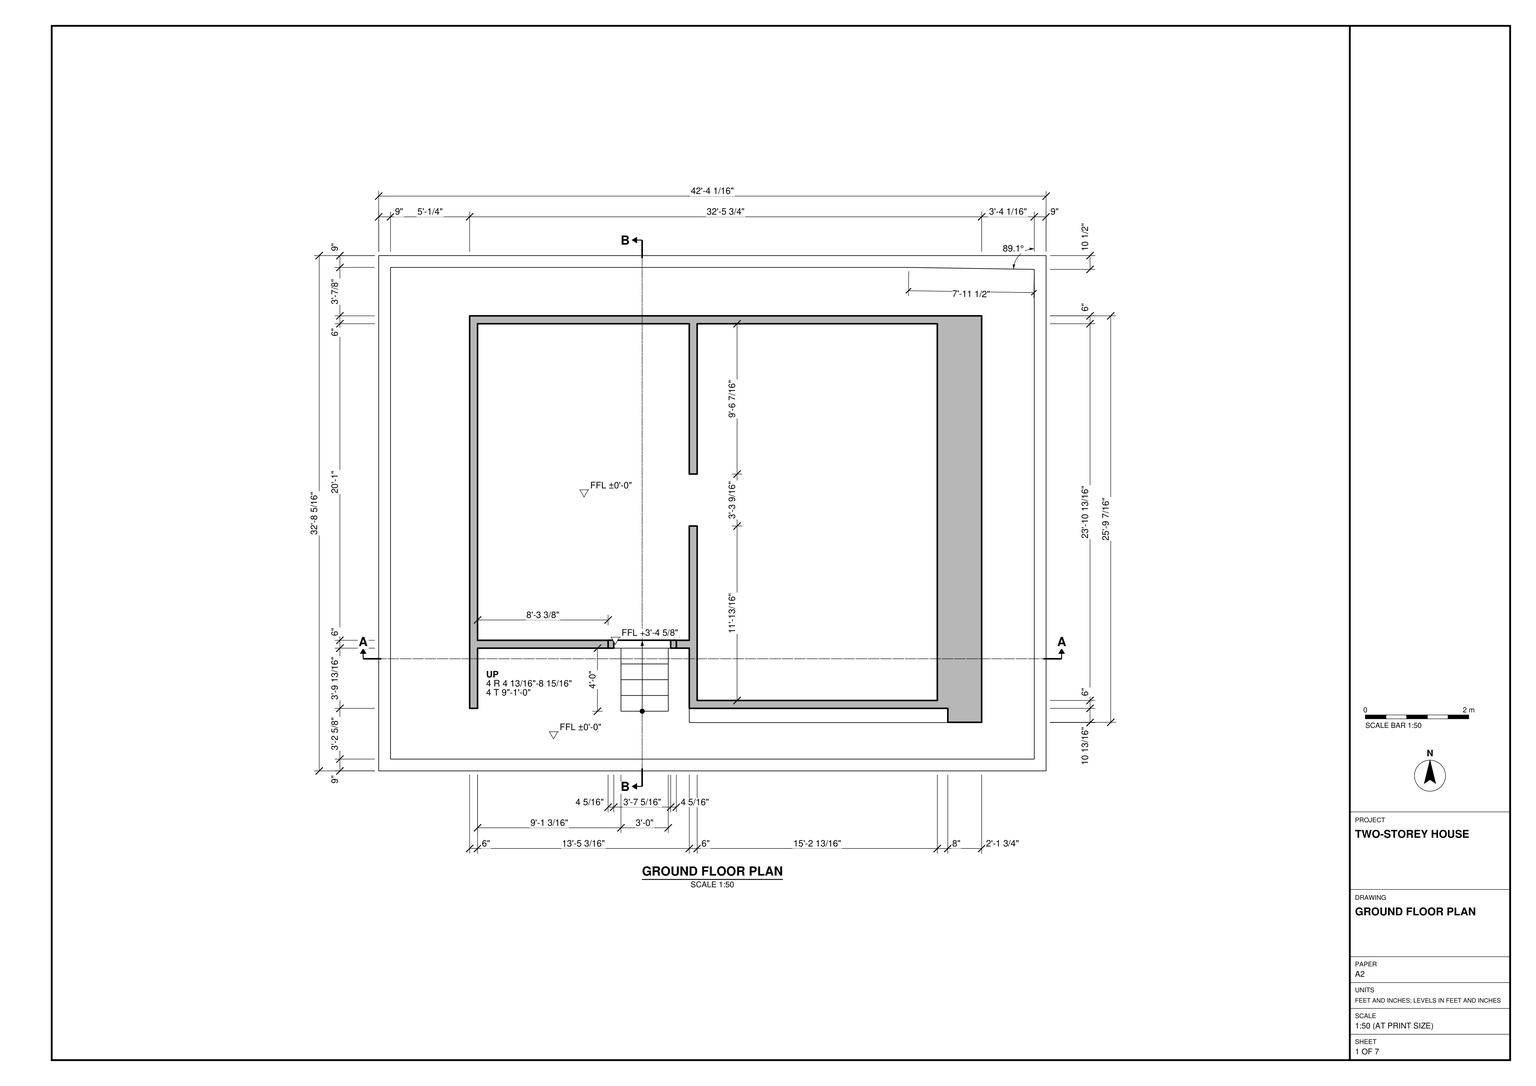
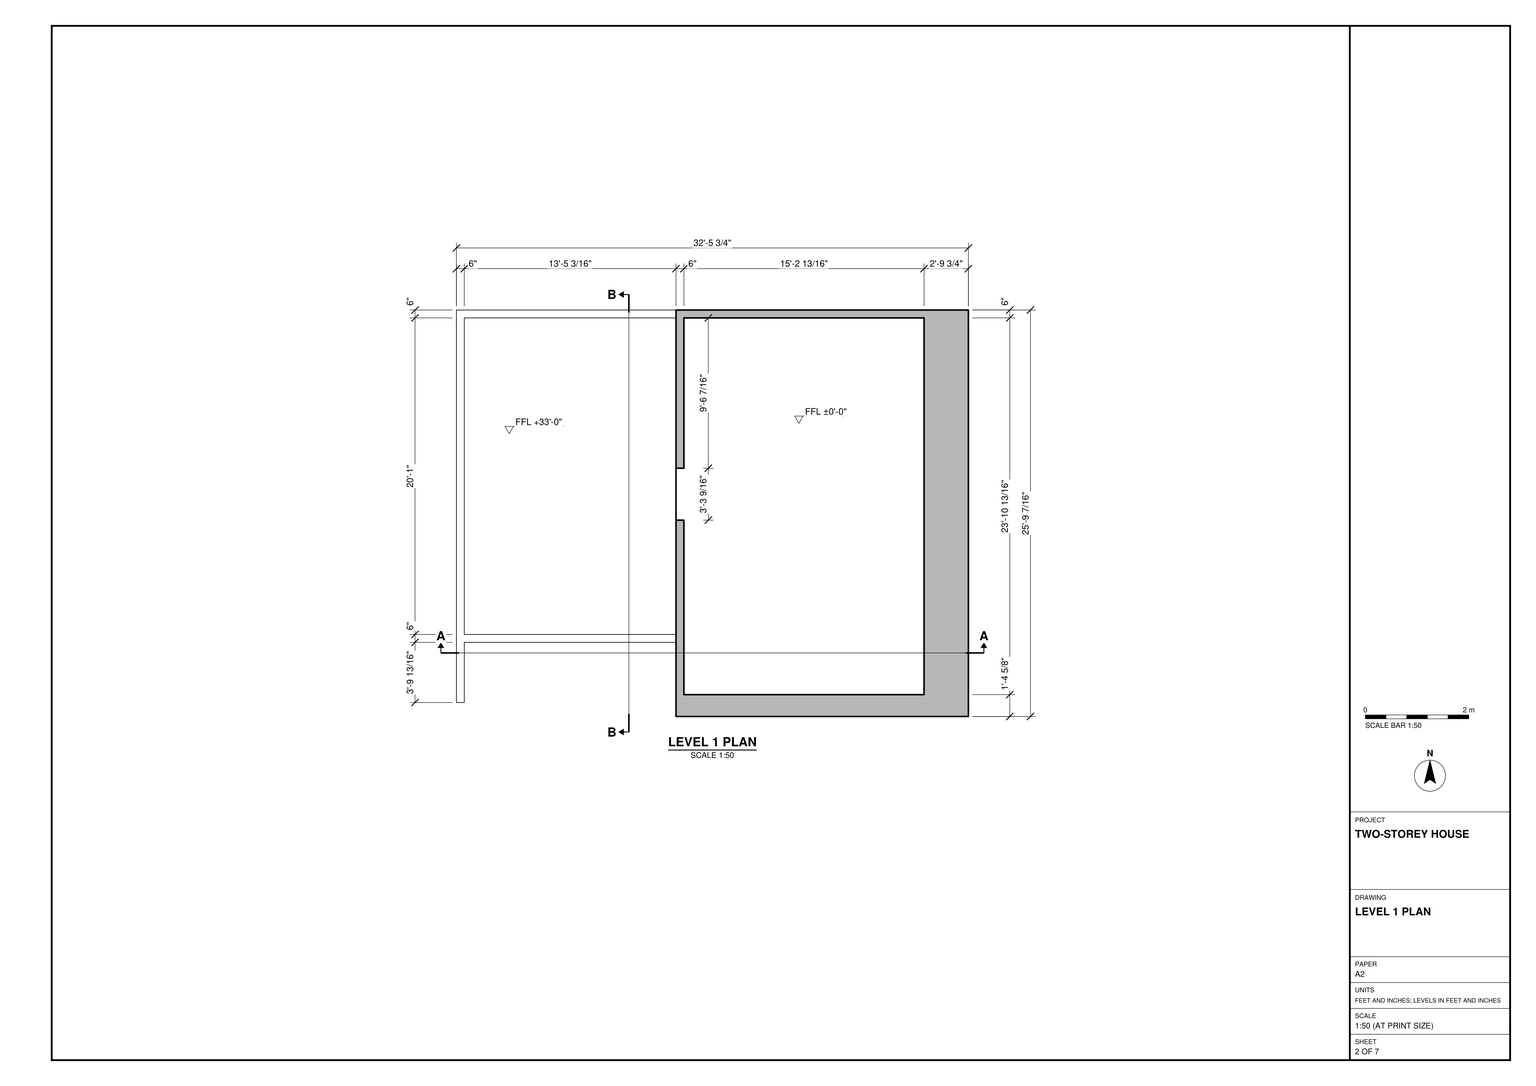
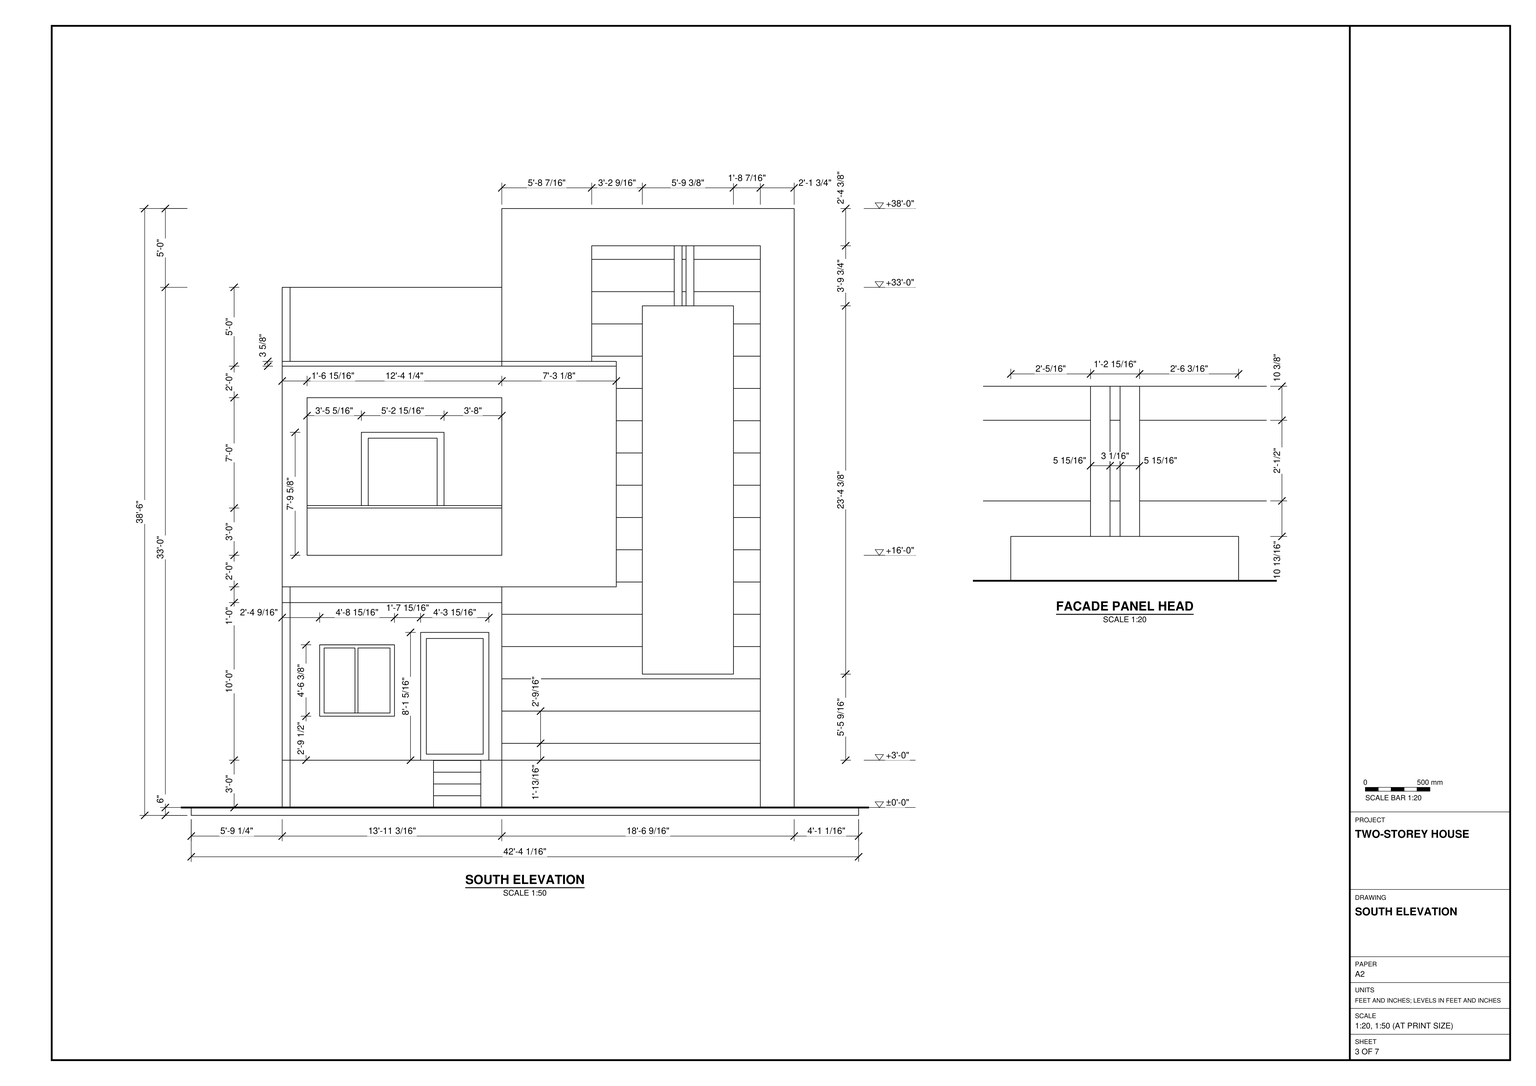
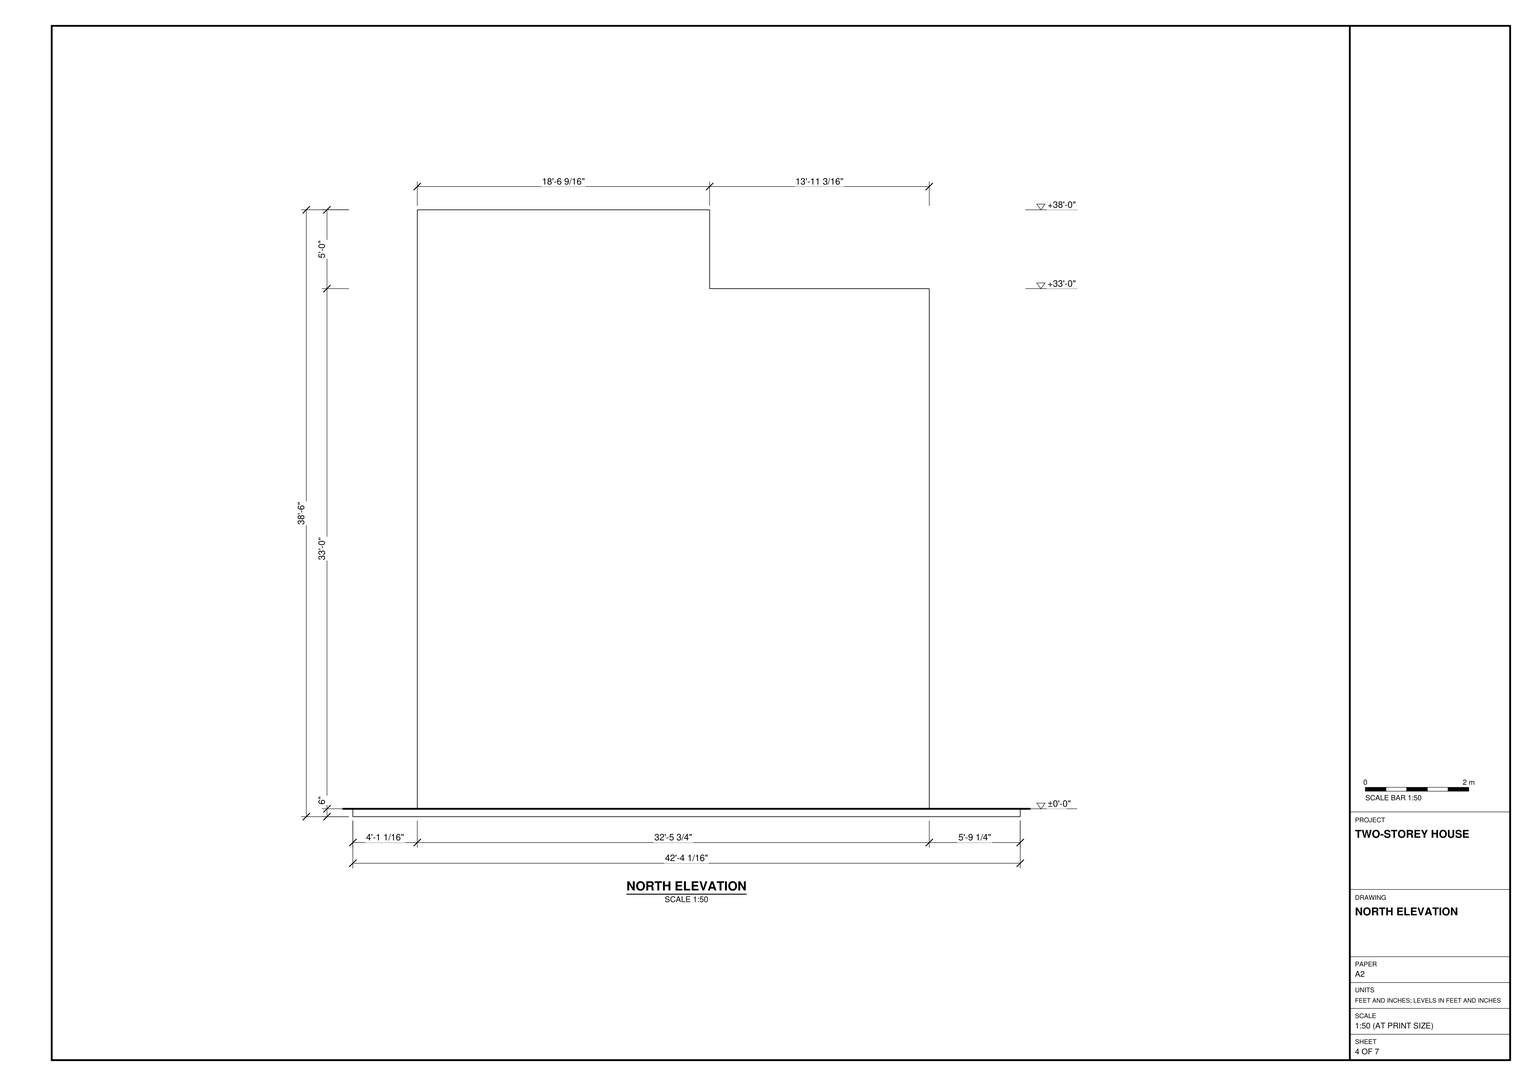
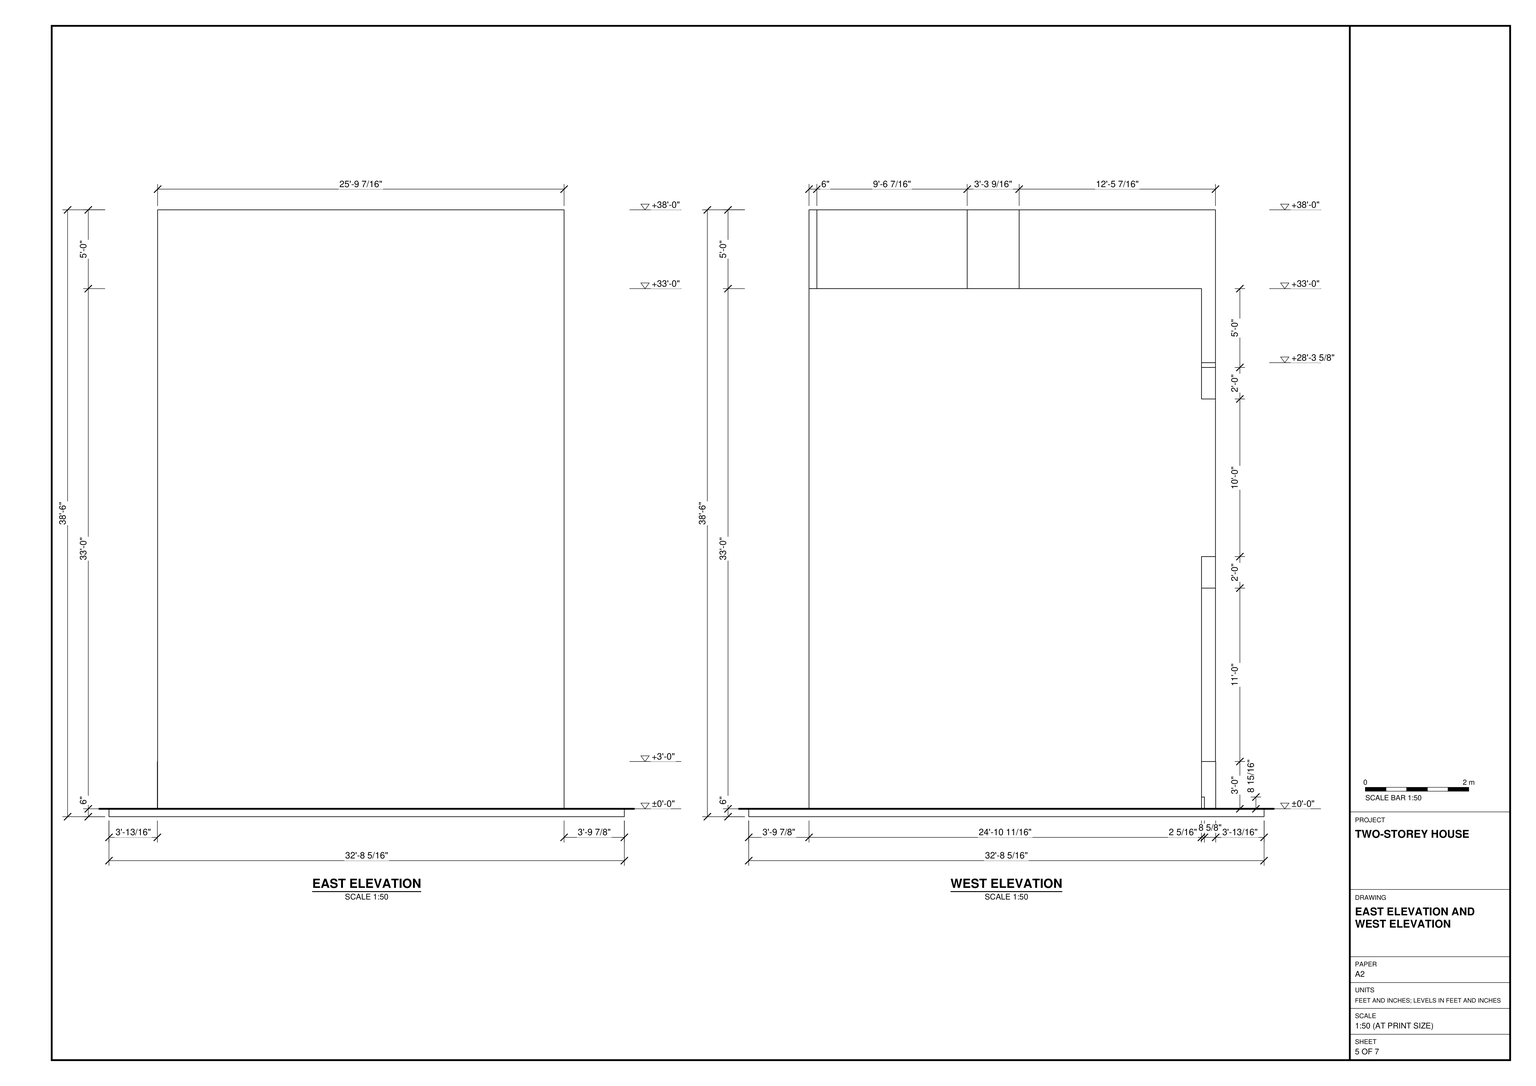
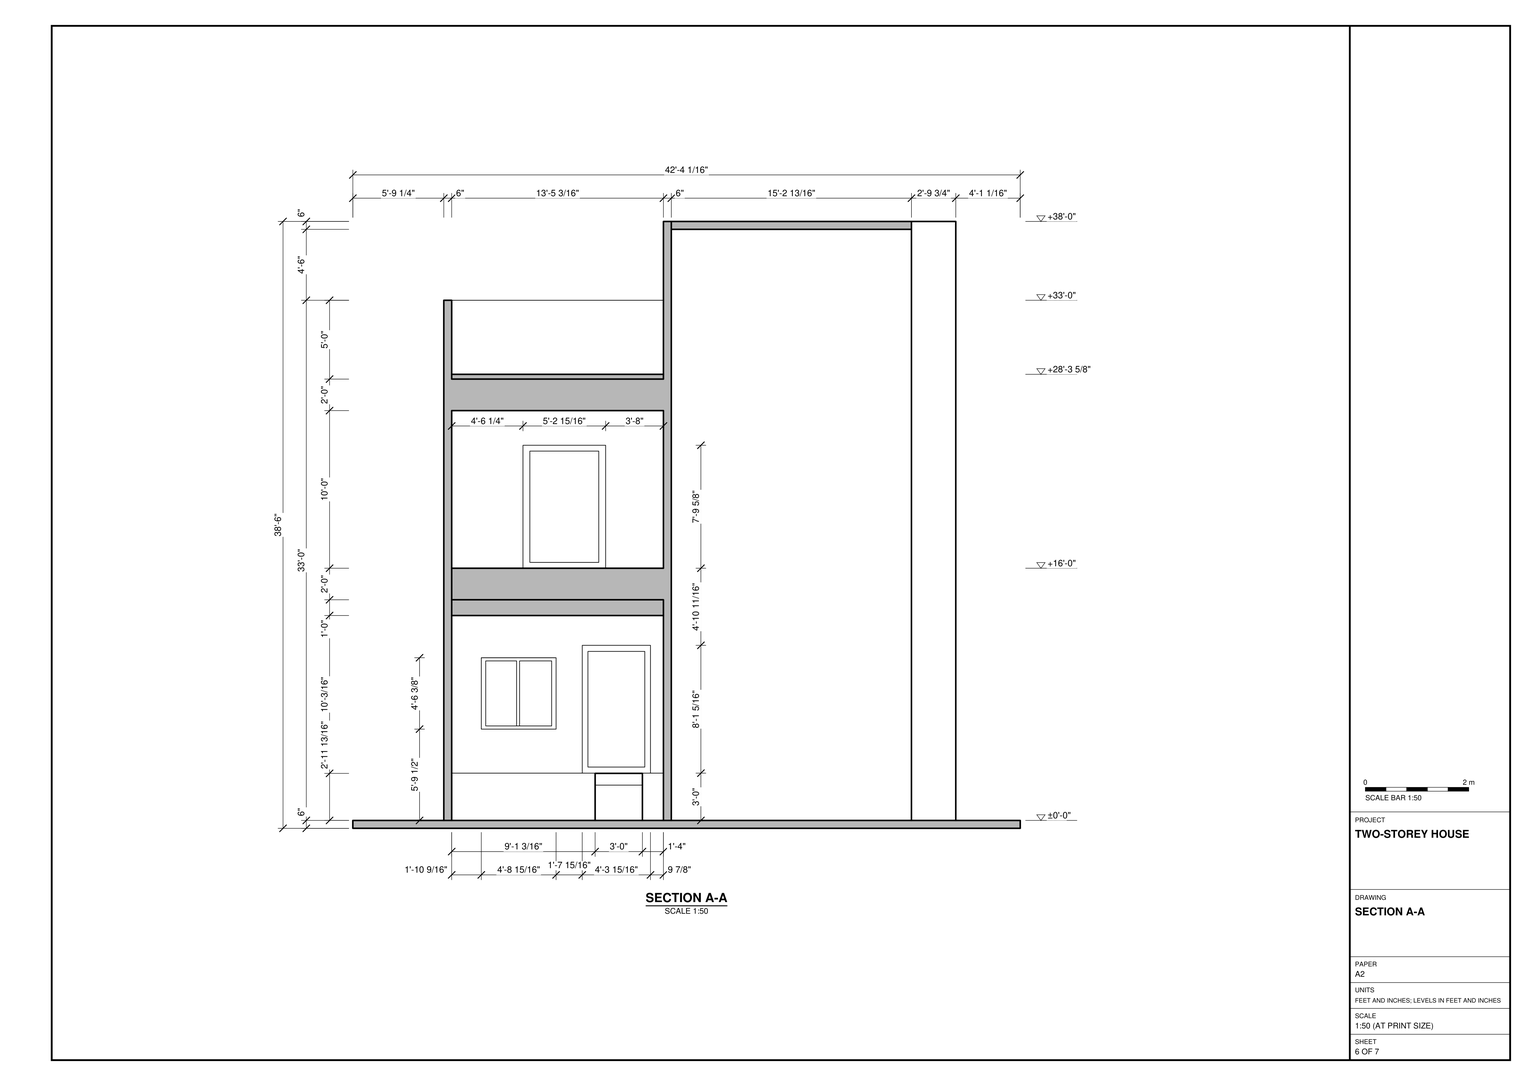
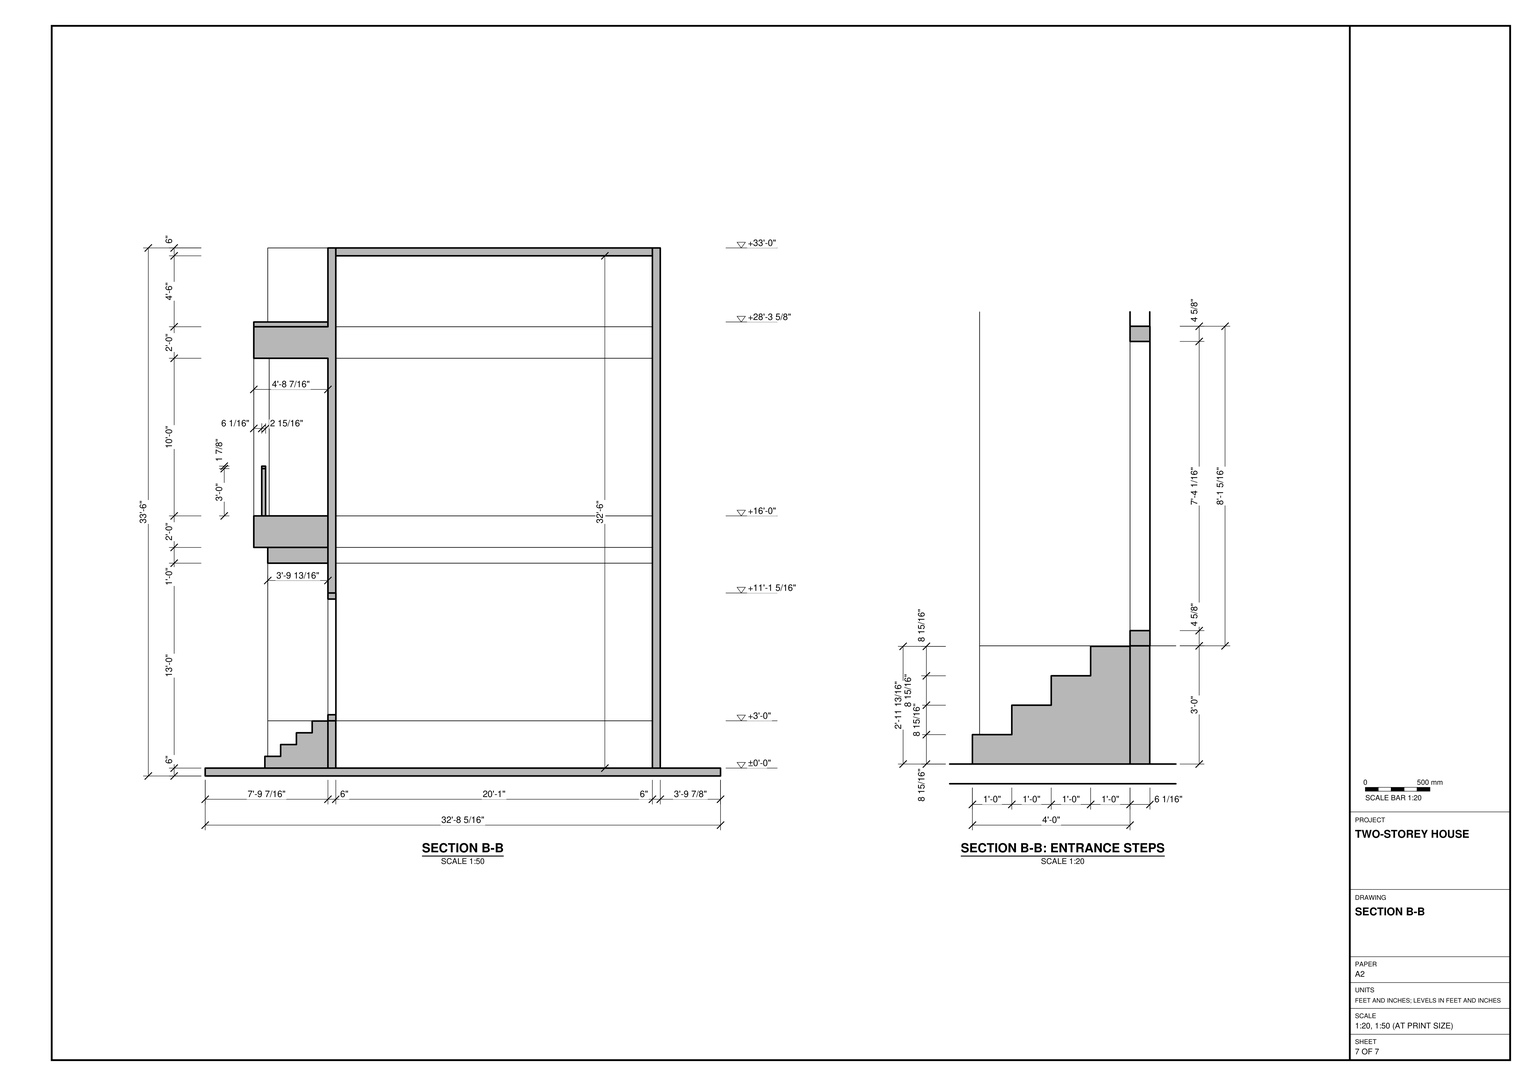
Build the house in SketchUp from task_files/diagram_01.pdf. Work in feet and inches. Including the base slab, the model measures 42'-4 1/16" along X, 32'-8 5/16" along Y and 38'-6" along Z. Use ±0'-0" for the ground-floor datum and +33'-0" for the upper level marked on the plan.

Set out the house on the base slab using the offsets on the ground-floor plan. Model the exterior walls and central dividing wall at their drawn thicknesses, including the passage between the two bays. Follow the level plan for the extent of the upper slab and the elevation for the stepped roofline. On the south side, build the straight entrance steps up to the recessed doorway and place the divided window to its left. Above the entrance bay, model the broad rectangular frame around the recessed upper opening. On the taller bay, model the horizontal bands, the tall rectangular façade panel and the narrow vertical strips visible above its head.

Keep walls, slabs, roof elements and any furniture or joinery pieces shown as separate groups or components. Use components for repeated parts. Any decor or loose items shown may use suitable library components. Save one SketchUp model as output_files/two_storey_house_with_stepped_south_facade.skp.

# SketchUp Ruby script. Lengths in inches.
U = 1.inch
M = Sketchup.active_model
def pt(a) = Geom::Point3d.new(a.map { |v| v * U })
def face(e, loops, mat)
  f = e.add_face(loops[0].map { |a| pt(a) })
  loops[1..].each { |l| e.add_face(l.map { |a| pt(a) }).erase! }
  f.material = f.back_material = mat if mat
  f
end
# faces: each face lists its corners as indices into pts; further lists are holes
def faces(e, pts, list, mat = nil) = list.each { |f| face(e, (f[0].is_a?(Array) ? f : [f]).map { |l| l.map { |i| pts[i] } }, mat) }
# xy, xz, yz: faces in a plane at the given z, y or x. An outline is a flat list of corners, or four numbers for a rectangle; further outlines are holes
def ring(l) = l.size == 4 ? [[l[0], l[1]], [l[2], l[1]], [l[2], l[3]], [l[0], l[3]]] : l.each_slice(2).to_a
def flat(e, list, mat, &to3) = list.each { |f| face(e, (f[0].is_a?(Array) ? f : [f]).map { |l| ring(l).map { |u, v| to3.(u, v) } }, mat) }
def xy(e, z, list, mat = nil) = flat(e, list, mat) { |x, y| [x, y, z] }
def xz(e, y, list, mat = nil) = flat(e, list, mat) { |x, z| [x, y, z] }
def yz(e, x, list, mat = nil) = flat(e, list, mat) { |y, z| [x, y, z] }
def lines(e, pts, list) = list.each { |a, b| e.add_line(pt(pts[a]), pt(pts[b])) }
# prism: a flat outline (further loops are holes) pulled along v
def prism(e, loops, v, mat = nil)
  f = face(e, loops, mat); d = Geom::Vector3d.new(v.map { |x| x * U })
  f.pushpull(f.normal.samedirection?(d) ? d.length : -d.length)
end
def box(e, o, s, mat = nil) = prism(e, [[o, [o[0] + s[0], o[1], o[2]], [o[0] + s[0], o[1] + s[1], o[2]], [o[0], o[1] + s[1], o[2]]]], [0, 0, s[2]], mat)
def at(x, y, z, deg = 0) = Geom::Transformation.translation(pt([x, y, z])) * Geom::Transformation.rotation(ORIGIN, Z_AXIS, deg.degrees)
def axes(o, x, y, z) = Geom::Transformation.new([*x, 0, *y, 0, *z, 0, *pt(o).to_a, 1])
def part(name) = M.definitions.add(name)
# library, detail: a bought-in or finely detailed component or shape, given as its bounding box
def library(name, o, s) = part(name).tap { |d| box(d.entities, o, s) }
def detail(e, o, s) = box(e.add_group.entities, o, s)
def put(e, d, t, mat = nil) = e.add_instance(d, t).tap { |i| i.material = mat if mat }
def group(e, t, mat = nil) = e.add_group.tap { |g| g.transformation = t; g.material = mat if mat }.entities
root = M.entities
M.materials.add("[0035_Tan]").color = [210, 180, 140]
M.materials.add("[0043_SaddleBrown]").color = [139, 69, 19]
M.materials.add("[0050_LemonChiffon]").color = [255, 250, 205]
M.materials.add("[0119_RosyBrown]").color = [188, 143, 143]
M.materials.add("[0132_LightGray]").color = [169, 169, 169]
M.materials.add("[0134_DimGray]").color = [105, 105, 105]
M.materials.add("[Color D07]").color = [153, 114, 0]
M.materials.add("[Color D08]").color = [102, 76, 0]
M.materials.add("[Color E02]").color = [255, 255, 153]
M.materials.add("[Color E07]").color = [153, 153, 119]
M.materials.add("[Metal Seamed]").color = [118, 119, 115]
M.materials.add("[Stone Marble]").color = [143, 138, 136]
M.materials.add("[Translucent Glass Blue]").color = [100, 149, 237]
M.materials["[Translucent Glass Blue]"].alpha = 0.5
M.materials.add("[Translucent Glass Gray]").color = [128, 128, 128]
M.materials["[Translucent Glass Gray]"].alpha = 0.5
c1 = part("Group\#2")
xy(c1.entities,0,[[0,0,48,6.0625]],"[0043_SaddleBrown]")
xy(c1.entities,4,[[4,0,44,6.0625]],"[0043_SaddleBrown]")
xy(c1.entities,80,[[4,0,44,6.0625]])
xy(c1.entities,84,[[0,0,48,6.0625]],"[0043_SaddleBrown]")
xz(c1.entities,0,[[[0,0,48,84],[4,4,44,80]]],"[0043_SaddleBrown]")
xz(c1.entities,6.0625,[[[0,0,48,84],[4,4,44,80]],[4,4,44,80]],"[0043_SaddleBrown]")
yz(c1.entities,0,[[0,0,6.0625,84]],"[0043_SaddleBrown]")
yz(c1.entities,4,[[0,4,6.0625,80]],"[0043_SaddleBrown]")
yz(c1.entities,44,[[0,4,6.0625,80]],"[0043_SaddleBrown]")
yz(c1.entities,48,[[0,0,6.0625,84]],"[0043_SaddleBrown]")
xy(root,0,[[0,0,508.0625,392.3125]])
xy(root,6,[[[0,0,508.0625,392.3125],[9,9,9,383.3125,403.5625,383.3125,499.0625,381.8125,499.0625,9]],[[9,9,499.0625,9,499.0625,381.8125,403.5625,383.3125,9,383.3125],[236.4375,36.8125,236.4375,93.4375,220.44,93.4375,220.44,45.4375,184.44,45.4375,184.44,93.4375,75.25,93.4375,75.25,47.625,69.25,47.625,69.25,346.4375,459,346.4375,459,37,433.25,37,433.25,36.8125]],[236.4375,36.8125,433.25,47.625],[433.25,37,459,346.4375],[184.44,45.4375,220.44,57.4375],
  [[69.25,47.625,69.25,346.4375,433.25,346.4375,433.25,47.625,236.4375,47.625,236.4375,93.4375,75.25,93.4375,75.25,47.625],[242.4375,53.625,425.25,53.625,425.25,340.4375,242.4375,340.4375,242.4375,226,236.4375,226,236.4375,340.4375,75.25,340.4375,75.25,99.4375,236.4375,99.4375,236.4375,186.46,242.4375,186.46]],[242.4375,53.625,425.25,53.625,425.25,340.4375,242.4375,340.4375,242.4375,226,236.4375,226,236.4375,340.4375,75.25,340.4375,75.25,99.4375,236.4375,99.4375,236.4375,186.46,242.4375,186.46],[184.44,57.4375,220.44,93.4375]])
xy(root,14.96,[[184.44,45.4375,220.44,57.4375]],"[0119_RosyBrown]")
xy(root,23.92,[[184.44,57.4375,220.44,69.4375]],"[0119_RosyBrown]")
xy(root,32.88,[[184.44,69.4375,220.44,81.4375]],"[0119_RosyBrown]")
xy(root,41.84,[[184.44,81.4375,220.44,93.4375]],"[0119_RosyBrown]")
xy(root,42,[[174.64,93.4375,226.58,99.4375]])
xy(root,42,[[236.4375,36.8125,433.25,47.625]],"[Stone Marble]")
xy(root,75.51,[[97.79,93.4375,154.72,99.4375]])
xy(root,107.55,[[343.41,47.625,412.79,53.625]])
xy(root,129.82,[[97.79,93.4375,154.72,99.4375]])
xy(root,139.3125,[[174.64,93.4375,226.58,99.4375]])
xy(root,162,[[75.25,47.625,236.4375,93.4375]])
xy(root,174,[[69.25,37,236.4375,47.625],[236.4375,37,323.59,47.625],[75.25,47.625,236.4375,93.4375]])
xy(root,198,[[88.1875,43.0625,236.4375,46],[88.1875,46,236.4375,46,236.4375,93.4375,75.25,93.4375,75.25,48.72,88.1875,48.72],[129.51,93.4375,192.45,99.4375]])
xy(root,198,[[88.1875,37,236.4375,43.0625]],"[0134_DimGray]")
xy(root,234,[[88.1875,43.0625,236.4375,46]],"[Metal Seamed]")
xy(root,235.875,[[88.1875,43.0625,236.4375,46]],"[Metal Seamed]")
xy(root,291.625,[[129.51,93.4375,192.45,99.4375]])
xy(root,318,[[88.1875,37,88.1875,48.72,75.25,48.72,75.25,93.4375,236.4375,93.4375,236.4375,37]])
xy(root,342,[[69.25,37,69.25,47.625,75.25,47.625,75.25,93.4375,236.4375,93.4375,236.4375,37],[236.4375,37,323.59,47.625]])
xy(root,345.625,[[69.25,37,236.4375,37,236.4375,93.4375,75.25,93.4375,75.25,47.625,69.25,47.625],[236.4375,37,304.875,47.625],[304.875,37,323.59,47.625]])
xy(root,387.92,[[343.41,47.625,412.79,53.625]])
xy(root,387.92,[[367.69,43.125,373.64,47.625],[376.69,43.125,382.64,47.625]],"[Color E02]")
xy(root,396,[[75.25,99.4375,236.4375,340.4375]])
xy(root,402,[[69.25,47.625,75.25,47.625,75.25,93.4375,236.4375,93.4375,236.4375,99.4375,75.25,99.4375,75.25,340.4375,236.4375,340.4375,236.4375,346.4375,69.25,346.4375],[75.25,99.4375,236.4375,340.4375]])
xy(root,433.64,[[304.875,37,304.875,47.625,367.69,47.625,367.69,43.125,373.64,43.125,373.64,47.625,376.69,47.625,376.69,43.125,382.64,43.125,382.64,47.625,433.25,47.625,433.25,37]],"[Color D07]")
xy(root,433.64,[[367.69,43.125,373.64,47.625],[376.69,43.125,382.64,47.625]],"[Color E02]")
xy(root,456,[[242.4375,53.625,425.25,340.4375]])
xy(root,462,[[236.4375,37,433.25,37,433.25,346.4375,236.4375,346.4375,236.4375,226,242.4375,226,242.4375,340.4375,425.25,340.4375,425.25,53.625,242.4375,53.625,242.4375,186.46,236.4375,186.46],[433.25,37,459,346.4375],[242.4375,53.625,425.25,340.4375],[236.4375,186.46,242.4375,226]])
xz(root,0,[[0,0,508.0625,6]])
xz(root,36.8125,[[236.4375,6,433.25,42]],"[Stone Marble]")
xz(root,37,[[69.25,342,236.4375,345.625],[236.4375,342,323.59,345.625]])
xz(root,37,[[[69.25,174,323.59,342],[88.1875,198,236.4375,318]]],"[0134_DimGray]")
xz(root,37,[[433.25,6,459,6,459,462,236.4375,462,236.4375,345.625,304.875,345.625,304.875,433.64,433.25,433.64]],"[Color D08]")
xz(root,43.0625,[[88.1875,234,236.4375,235.875]],"[Metal Seamed]")
xz(root,43.0625,[[88.1875,198,236.4375,234]],"[Translucent Glass Blue]")
xz(root,43.125,[[367.69,387.92,373.64,433.64],[376.69,387.92,382.64,433.64]],"[Color E02]")
xz(root,45.4375,[[184.44,6,220.44,14.96]],"[0119_RosyBrown]")
xz(root,46,[[88.1875,234,236.4375,235.875]],"[Metal Seamed]")
xz(root,46,[[88.1875,198,236.4375,234]],"[Translucent Glass Blue]")
xz(root,47.625,[[69.25,6,75.25,42],[236.4375,6,433.25,42],[69.25,42,75.25,162],[69.25,162,75.25,174],[75.25,162,236.4375,174],
  [69.25,174,75.25,198],[69.25,342,75.25,345.625],[236.4375,342,304.875,345.625],[304.875,342,323.59,345.625]])
xz(root,47.625,[[69.25,345.625,75.25,402]],"[0050_LemonChiffon]")
xz(root,47.625,[[367.69,387.92,373.64,398.72],[376.69,387.92,382.64,398.72],[367.69,398.72,373.64,423.28],[376.69,398.72,382.64,423.28],[367.69,423.28,373.64,433.64],
  [376.69,423.28,382.64,433.64]],"[Color E02]")
xz(root,47.625,[[236.4375,42,433.25,54.84],[236.4375,54.84,433.25,79.41],[236.4375,79.41,433.25,103.97],[236.4375,103.97,433.25,103.97,433.25,128.53,412.79,128.53,412.79,107.55,343.41,107.55,343.41,128.53,236.4375,128.53],[236.4375,128.53,343.41,153.09],
  [412.79,128.53,433.25,153.09],[236.4375,153.09,343.41,153.09,343.41,177.66,323.59,177.66,323.59,174,236.4375,174],[412.79,153.09,433.25,177.66],[323.59,177.66,343.41,202.22],[412.79,177.66,433.25,202.22],
  [323.59,202.22,343.41,226.78],[412.79,202.22,433.25,226.78],[323.59,226.78,343.41,251.34],[412.79,226.78,433.25,251.34],[323.59,251.34,343.41,275.91],
  [412.79,251.34,433.25,275.91],[323.59,275.91,343.41,300.47],[412.79,275.91,433.25,300.47],[323.59,300.47,343.41,325.03],[412.79,300.47,433.25,325.03],
  [323.59,325.03,343.41,325.03,343.41,349.59,304.875,349.59,304.875,345.625,323.59,345.625],[412.79,325.03,433.25,349.59],[304.875,349.59,343.41,374.16],[412.79,349.59,433.25,374.16],[304.875,374.16,343.41,374.16,343.41,387.92,367.69,387.92,367.69,398.72,304.875,398.72],
  [412.79,374.16,433.25,374.16,433.25,398.72,382.64,398.72,382.64,387.92,412.79,387.92],[373.64,387.92,376.69,398.72],[304.875,398.72,367.69,423.28],[373.64,398.72,376.69,423.28],[382.64,398.72,433.25,423.28],
  [304.875,423.28,367.69,433.64],[373.64,423.28,376.69,433.64],[382.64,423.28,433.25,433.64]],"[Color E07]")
xz(root,48.72,[[75.25,198,88.1875,318]])
xz(root,53.625,[[[242.4375,6,425.25,456],[343.41,107.55,412.79,387.92]],[242.4375,456,425.25,462]])
xz(root,53.625,[[343.41,107.55,412.79,387.92]],"[Translucent Glass Gray]")
xz(root,57.4375,[[184.44,14.96,220.44,23.92]],"[0119_RosyBrown]")
xz(root,69.4375,[[184.44,23.92,220.44,32.88]],"[0119_RosyBrown]")
xz(root,81.4375,[[184.44,32.88,220.44,41.84]],"[0119_RosyBrown]")
xz(root,93.4375,[[184.44,6,220.44,32.88],[184.44,32.88,220.44,41.84],[75.25,162,236.4375,174],[75.25,174,236.4375,198],[75.25,342,236.4375,345.625]])
xz(root,93.4375,[[75.25,198,129.51,198,129.51,291.625,192.45,291.625,192.45,198,236.4375,198,236.4375,318,75.25,318]],"[0035_Tan]")
xz(root,93.4375,[[75.25,345.625,236.4375,402]],"[0050_LemonChiffon]")
xz(root,93.4375,[[75.25,6,184.44,6,184.44,41.84,220.44,41.84,220.44,6,236.4375,6,236.4375,42,75.25,42],[[75.25,42,174.64,42,174.64,139.3125,226.58,139.3125,226.58,42,236.4375,42,236.4375,162,75.25,162],[97.79,75.51,154.72,129.82]]],"[0132_LightGray]")
xz(root,99.4375,[[75.25,6,236.4375,42],[[75.25,42,75.25,162,236.4375,162,236.4375,42,226.58,42,226.58,139.3125,174.64,139.3125,174.64,42],[97.79,75.51,154.72,129.82]],[75.25,162,236.4375,174],[75.25,174,236.4375,198],[75.25,198,75.25,318,236.4375,318,236.4375,198,192.45,198,192.45,291.625,129.51,291.625,129.51,198],
  [75.25,318,236.4375,342],[75.25,342,236.4375,396],[75.25,396,236.4375,402]])
xz(root,186.46,[[236.4375,6,242.4375,42],[236.4375,42,242.4375,162],[236.4375,162,242.4375,174],[236.4375,174,242.4375,198],[236.4375,198,242.4375,318],
  [236.4375,318,242.4375,342],[236.4375,342,242.4375,462]])
xz(root,226,[[236.4375,6,242.4375,42],[236.4375,42,242.4375,162],[236.4375,162,242.4375,174],[236.4375,174,242.4375,198],[236.4375,198,242.4375,318],
  [236.4375,318,242.4375,342],[236.4375,342,242.4375,462]])
xz(root,340.4375,[[75.25,6,236.4375,42],[242.4375,6,425.25,456],[75.25,42,236.4375,162],[75.25,162,236.4375,174],[75.25,174,236.4375,198],
  [75.25,198,236.4375,318],[75.25,318,236.4375,342],[75.25,342,236.4375,396],[75.25,396,236.4375,402],[242.4375,456,425.25,462]])
xz(root,346.4375,[[69.25,6,69.25,402,236.4375,402,236.4375,462,459,462,459,6]],"[0050_LemonChiffon]")
xz(root,392.3125,[[0,0,508.0625,6]])
yz(root,0,[[0,0,392.3125,6]])
yz(root,69.25,[[37,174,47.625,198],[37,318,47.625,342],[37,342,47.625,345.625]])
yz(root,69.25,[[47.625,6,47.625,198,37,198,37,318,47.625,318,47.625,402,346.4375,402,346.4375,6]],"[0050_LemonChiffon]")
yz(root,75.25,[[47.625,6,93.4375,42],[99.4375,6,340.4375,42],[47.625,42,93.4375,162],[99.4375,42,340.4375,162],[47.625,162,93.4375,174],
  [99.4375,162,340.4375,174],[47.625,174,93.4375,198],[99.4375,174,340.4375,198],[99.4375,198,340.4375,318],[99.4375,318,340.4375,342],
  [47.625,342,93.4375,345.625],[99.4375,342,340.4375,396],[99.4375,396,340.4375,402]])
yz(root,75.25,[[47.625,345.625,93.4375,402]],"[0050_LemonChiffon]")
yz(root,75.25,[[48.72,198,93.4375,318]],"[0134_DimGray]")
yz(root,88.1875,[[43.0625,198,46,234]])
yz(root,88.1875,[[37,198,43.0625,198,43.0625,235.875,46,235.875,46,198,48.72,198,48.72,318,37,318]],"[0134_DimGray]")
yz(root,88.1875,[[43.0625,234,46,235.875]],"[Metal Seamed]")
yz(root,97.79,[[93.4375,75.51,99.4375,129.82]])
yz(root,129.51,[[93.4375,198,99.4375,291.625]])
yz(root,154.72,[[93.4375,75.51,99.4375,129.82]])
yz(root,174.64,[[93.4375,42,99.4375,139.3125]])
yz(root,184.44,[[45.4375,6,45.4375,14.96,57.4375,14.96,57.4375,23.92,69.4375,23.92,69.4375,32.88,81.4375,32.88,81.4375,41.84,93.4375,41.84,93.4375,6]],"[0119_RosyBrown]")
yz(root,192.45,[[93.4375,198,99.4375,291.625]])
yz(root,220.44,[[45.4375,6,93.4375,6,93.4375,41.84,81.4375,41.84,81.4375,32.88,69.4375,32.88,69.4375,23.92,57.4375,23.92,57.4375,14.96,45.4375,14.96]],"[0119_RosyBrown]")
yz(root,226.58,[[93.4375,42,99.4375,139.3125]])
yz(root,236.4375,[[99.4375,6,186.46,42],[226,6,340.4375,42],[47.625,42,93.4375,162],[99.4375,42,186.46,162],[226,42,340.4375,162],
  [47.625,162,93.4375,174],[99.4375,162,186.46,174],[226,162,340.4375,174],[99.4375,174,186.46,198],[226,174,340.4375,198],
  [43.0625,198,46,234],[99.4375,198,186.46,318],[226,198,340.4375,318],[99.4375,318,186.46,342],[226,318,340.4375,342],
  [37,342,47.625,345.625],[47.625,342,93.4375,345.625],[99.4375,342,186.46,396],[226,342,340.4375,396],[99.4375,396,186.46,402],
  [186.46,396,226,402],[226,396,340.4375,402],[186.46,402,226,462],[226,402,340.4375,462],[340.4375,402,346.4375,462]])
yz(root,236.4375,[[37,345.625,37,462,186.46,462,186.46,402,93.4375,402,93.4375,345.625]],"[0050_LemonChiffon]")
yz(root,236.4375,[[37,198,37,318,93.4375,318,93.4375,198,46,198,46,235.875,43.0625,235.875,43.0625,198]],"[0134_DimGray]")
yz(root,236.4375,[[43.0625,234,46,235.875]],"[Metal Seamed]")
yz(root,236.4375,[[36.8125,6,47.625,42],[47.625,6,93.4375,42]],"[Stone Marble]")
yz(root,242.4375,[[53.625,6,186.46,42],[226,6,340.4375,42],[53.625,42,186.46,162],[226,42,340.4375,162],[53.625,162,186.46,174],
  [226,162,340.4375,174],[53.625,174,186.46,198],[226,174,340.4375,198],[53.625,198,186.46,318],[226,198,340.4375,318],
  [53.625,318,186.46,342],[226,318,340.4375,342],[53.625,342,186.46,456],[226,342,340.4375,456],[53.625,456,186.46,462],
  [186.46,456,226,462],[226,456,325.3125,462],[325.3125,456,331.4375,462],[331.4375,456,340.4375,462]])
yz(root,304.875,[[37,345.625,47.625,433.64]],"[Color D07]")
yz(root,323.59,[[37,174,47.625,342],[37,342,47.625,345.625]])
yz(root,343.41,[[47.625,107.55,53.625,387.92]])
yz(root,367.69,[[43.125,387.92,47.625,433.64]],"[Color E02]")
yz(root,373.64,[[43.125,387.92,47.625,433.64]],"[Color E02]")
yz(root,376.69,[[43.125,387.92,47.625,433.64]],"[Color E02]")
yz(root,382.64,[[43.125,387.92,47.625,433.64]],"[Color E02]")
yz(root,412.79,[[47.625,107.55,53.625,387.92]])
yz(root,425.25,[[53.625,6,340.4375,456],[53.625,456,318.1875,462],[318.1875,456,331.4375,462],[331.4375,456,340.4375,462]])
yz(root,433.25,[[36.8125,6,37,42],[37,6,47.625,42]])
yz(root,433.25,[[37,42,47.625,433.64]],"[Color D07]")
yz(root,459,[[37,6,346.4375,462]],"[0050_LemonChiffon]")
yz(root,508.0625,[[0,0,392.3125,6]])
p = [[75.25,37,198],[75.25,47.625,198],[220.44,81.4375,23.92],[184.44,81.4375,23.92],[220.44,69.4375,14.96],[184.44,69.4375,14.96],
  [236.4375,47.625,177.66],[323.59,47.625,177.66],[236.4375,47.625,202.22],[323.59,47.625,202.22],[236.4375,47.625,226.78],[323.59,47.625,226.78],
  [236.4375,47.625,251.34],[323.59,47.625,251.34],[236.4375,47.625,275.91],[323.59,47.625,275.91],[236.4375,47.625,300.47],[323.59,47.625,300.47],
  [236.4375,47.625,325.03],[323.59,47.625,325.03],[236.4375,47.625,349.59],[304.875,47.625,349.59],[236.4375,47.625,374.16],[304.875,47.625,374.16],
  [236.4375,47.625,398.72],[304.875,47.625,398.72],[236.4375,47.625,423.28],[304.875,47.625,423.28],[236.4375,47.625,447.84],[433.25,47.625,447.84]]
lines(root,p,[[0,1],[2,3],[4,5],[6,7],[8,9],[10,11],[12,13],[14,15],[16,17],[18,19],[20,21],[22,23],
  [24,25],[26,27],[28,29]])
put(root,c1,axes([174.64,93.4375,42],[1.08203,0,0],[0,1,0],[0,0,1.15848]))
g1 = group(root,at(97.79,93.4375,75.51))
xy(g1,0,[[0,0,56.9375,2.6875]],"[0043_SaddleBrown]")
xy(g1,2.43,[[26.88,0,29.16,2.6875]])
xy(g1,2.43,[[3.38,0,26.88,2.6875],[29.16,0,53.56,2.6875]],"[0043_SaddleBrown]")
xy(g1,51.9375,[[3.38,0,26.88,2.6875],[29.16,0,53.56,2.6875]])
xy(g1,54.36,[[0,0,56.9375,2.6875]],"[0043_SaddleBrown]")
xz(g1,0,[[[0,0,56.9375,54.36],[3.38,2.43,3.38,51.9375,26.88,51.9375,26.88,2.43,29.16,2.43,29.16,51.9375,53.56,51.9375,53.56,2.43]]],"[0043_SaddleBrown]")
xz(g1,2.6875,[[[0,0,56.9375,54.36],[3.38,2.43,53.56,2.43,53.56,51.9375,29.16,51.9375,29.16,2.43,26.88,2.43,26.88,51.9375,3.38,51.9375]]],"[0043_SaddleBrown]")
xz(g1,2.6875,[[3.38,2.43,26.88,51.9375],[29.16,2.43,53.56,51.9375]],"[Translucent Glass Gray]")
yz(g1,0,[[0,0,2.6875,54.36]],"[0043_SaddleBrown]")
yz(g1,3.38,[[0,2.43,2.6875,51.9375]],"[0043_SaddleBrown]")
yz(g1,26.88,[[0,2.43,2.6875,51.9375]],"[0043_SaddleBrown]")
yz(g1,29.16,[[0,2.43,2.6875,51.9375]],"[0043_SaddleBrown]")
yz(g1,53.56,[[0,2.43,2.6875,51.9375]],"[0043_SaddleBrown]")
yz(g1,56.9375,[[0,0,2.6875,54.36]],"[0043_SaddleBrown]")
put(root,c1,axes([129.51,93.86,198],[1.3112,0,0],[0,0.93,0],[0,0,1.11458]))
